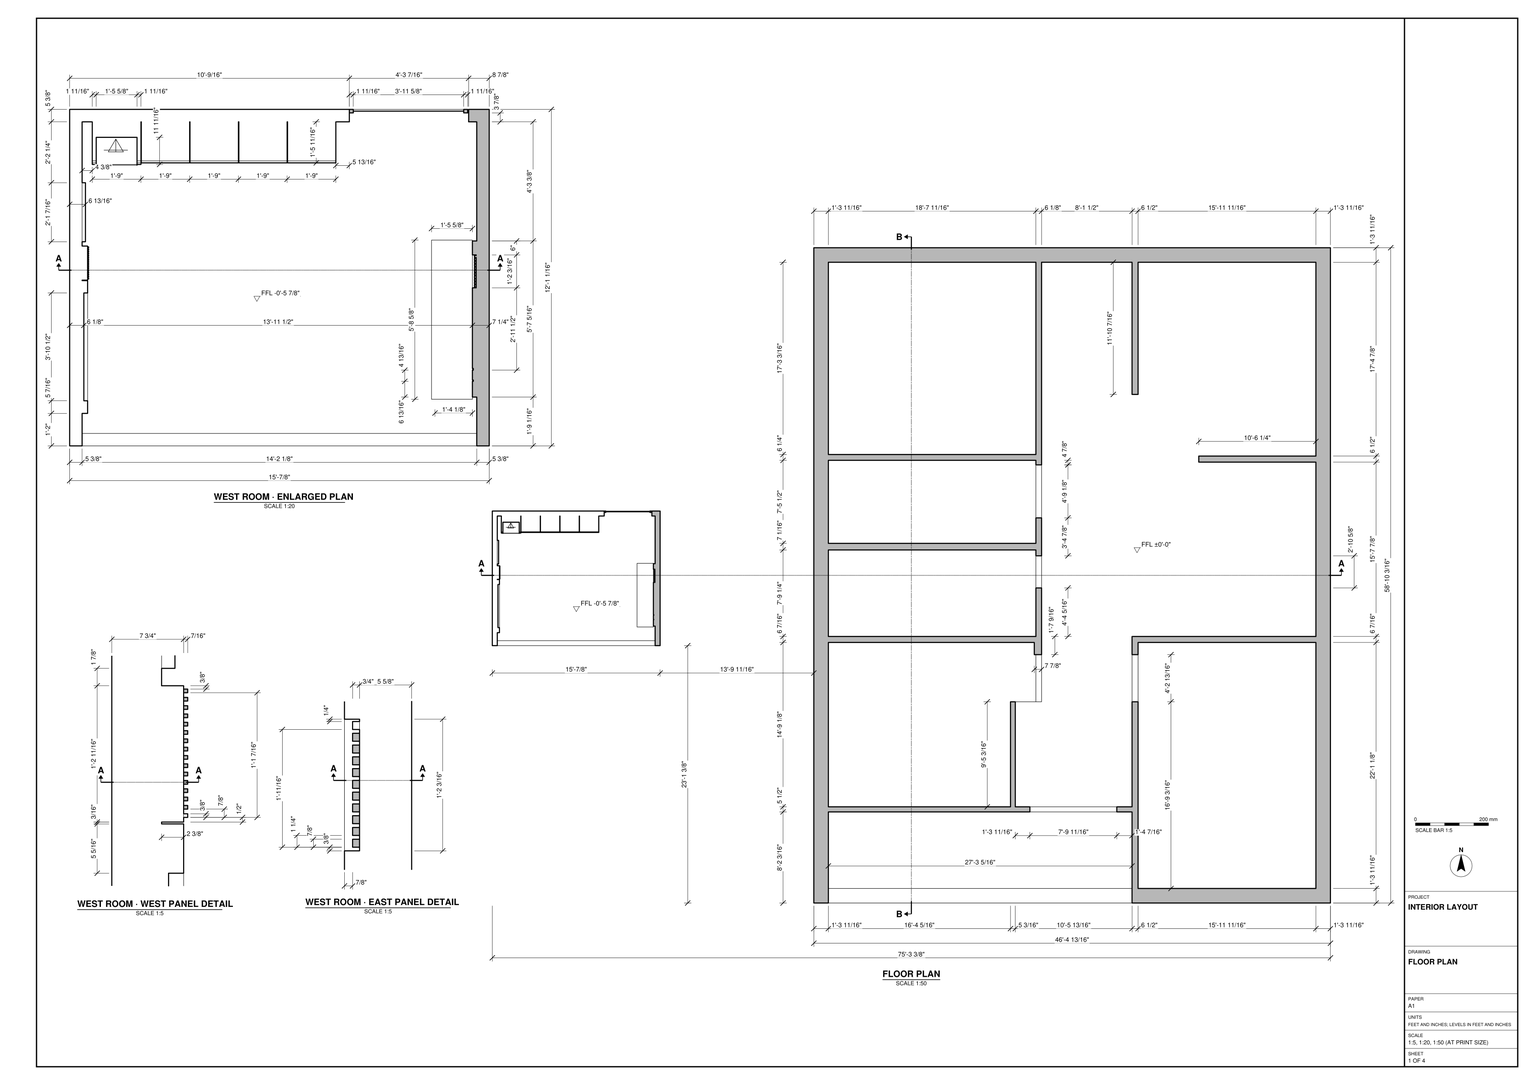
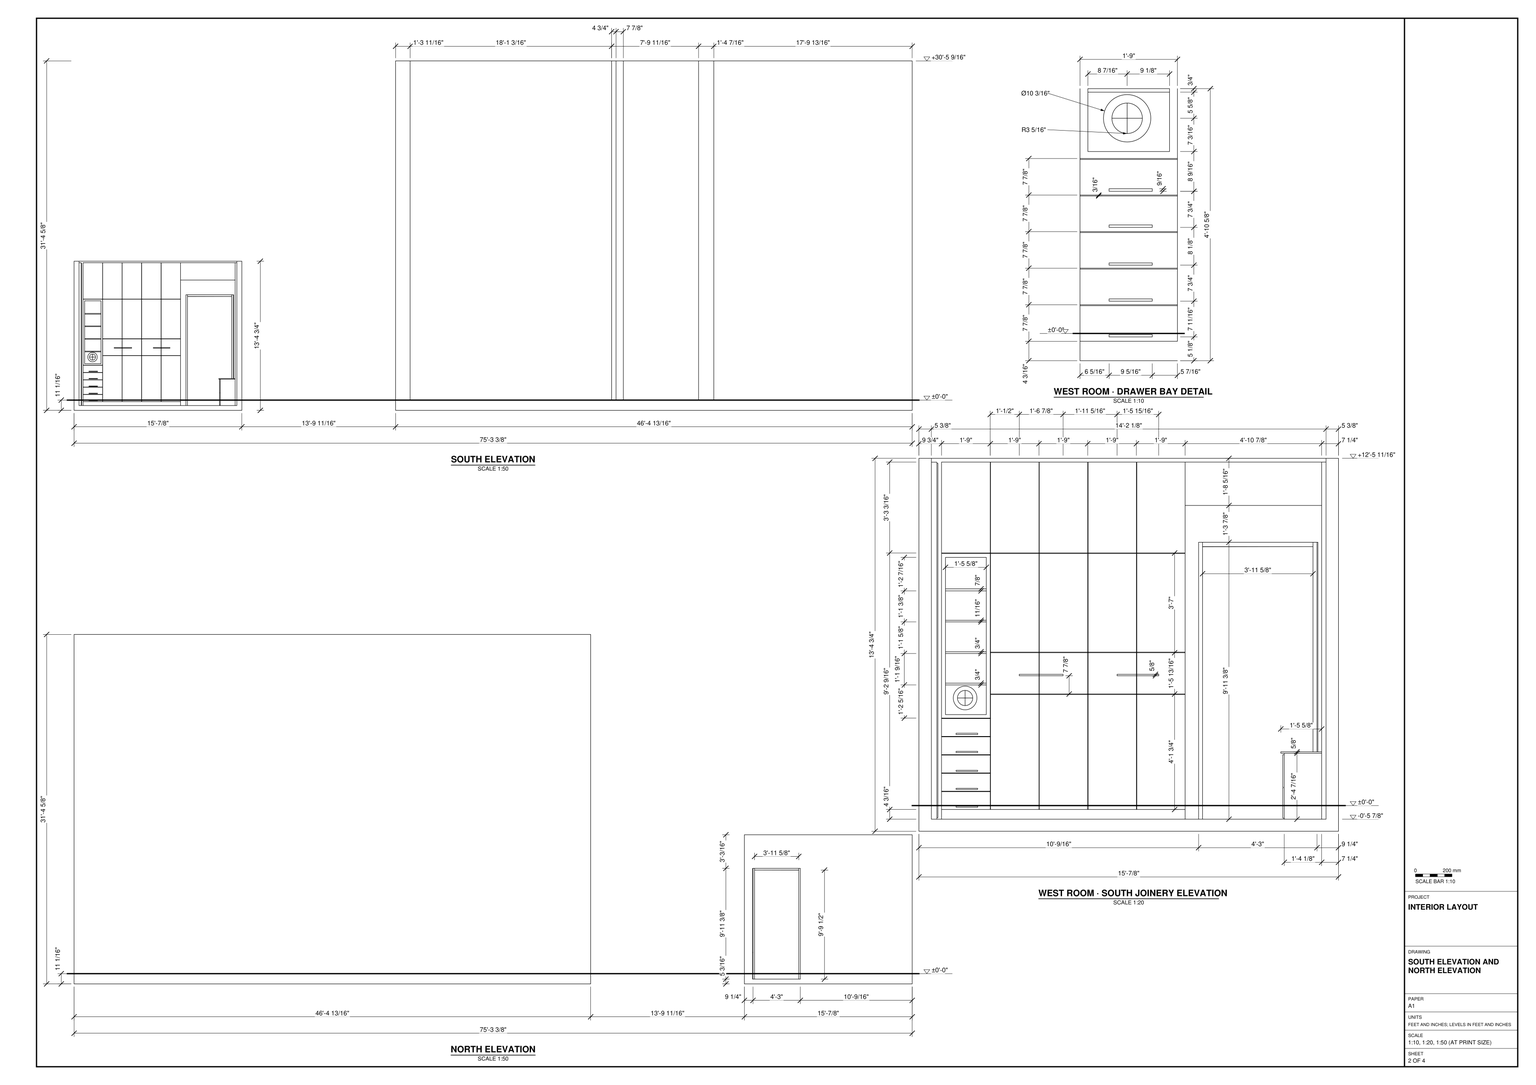
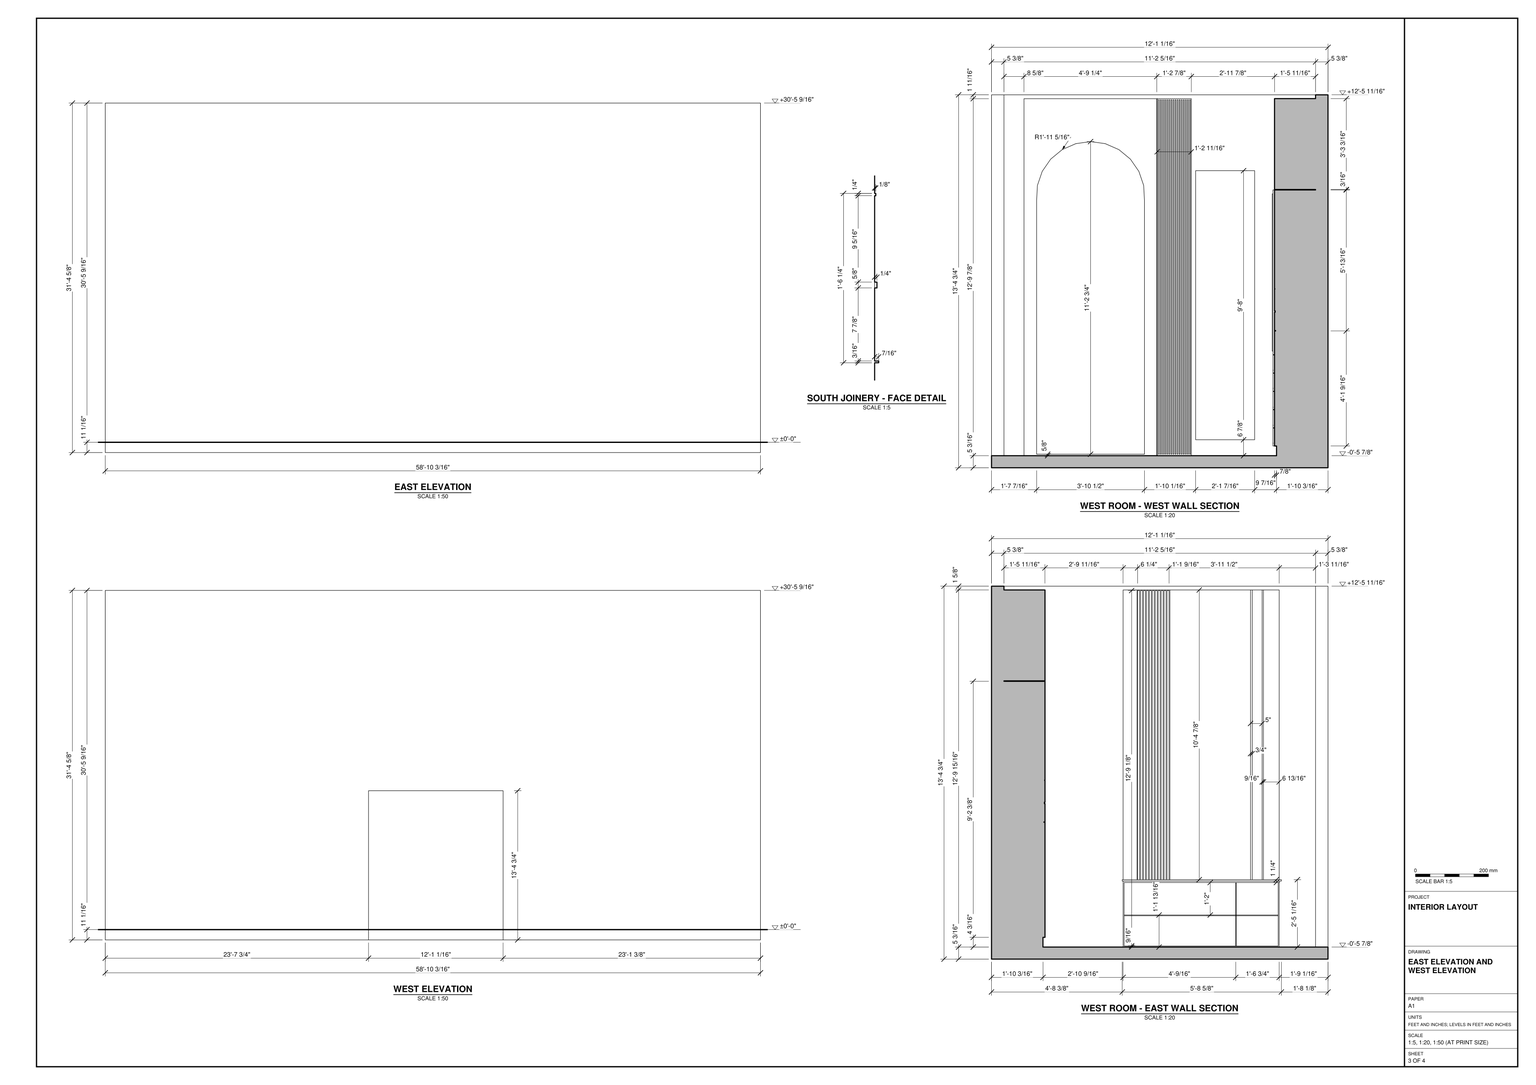
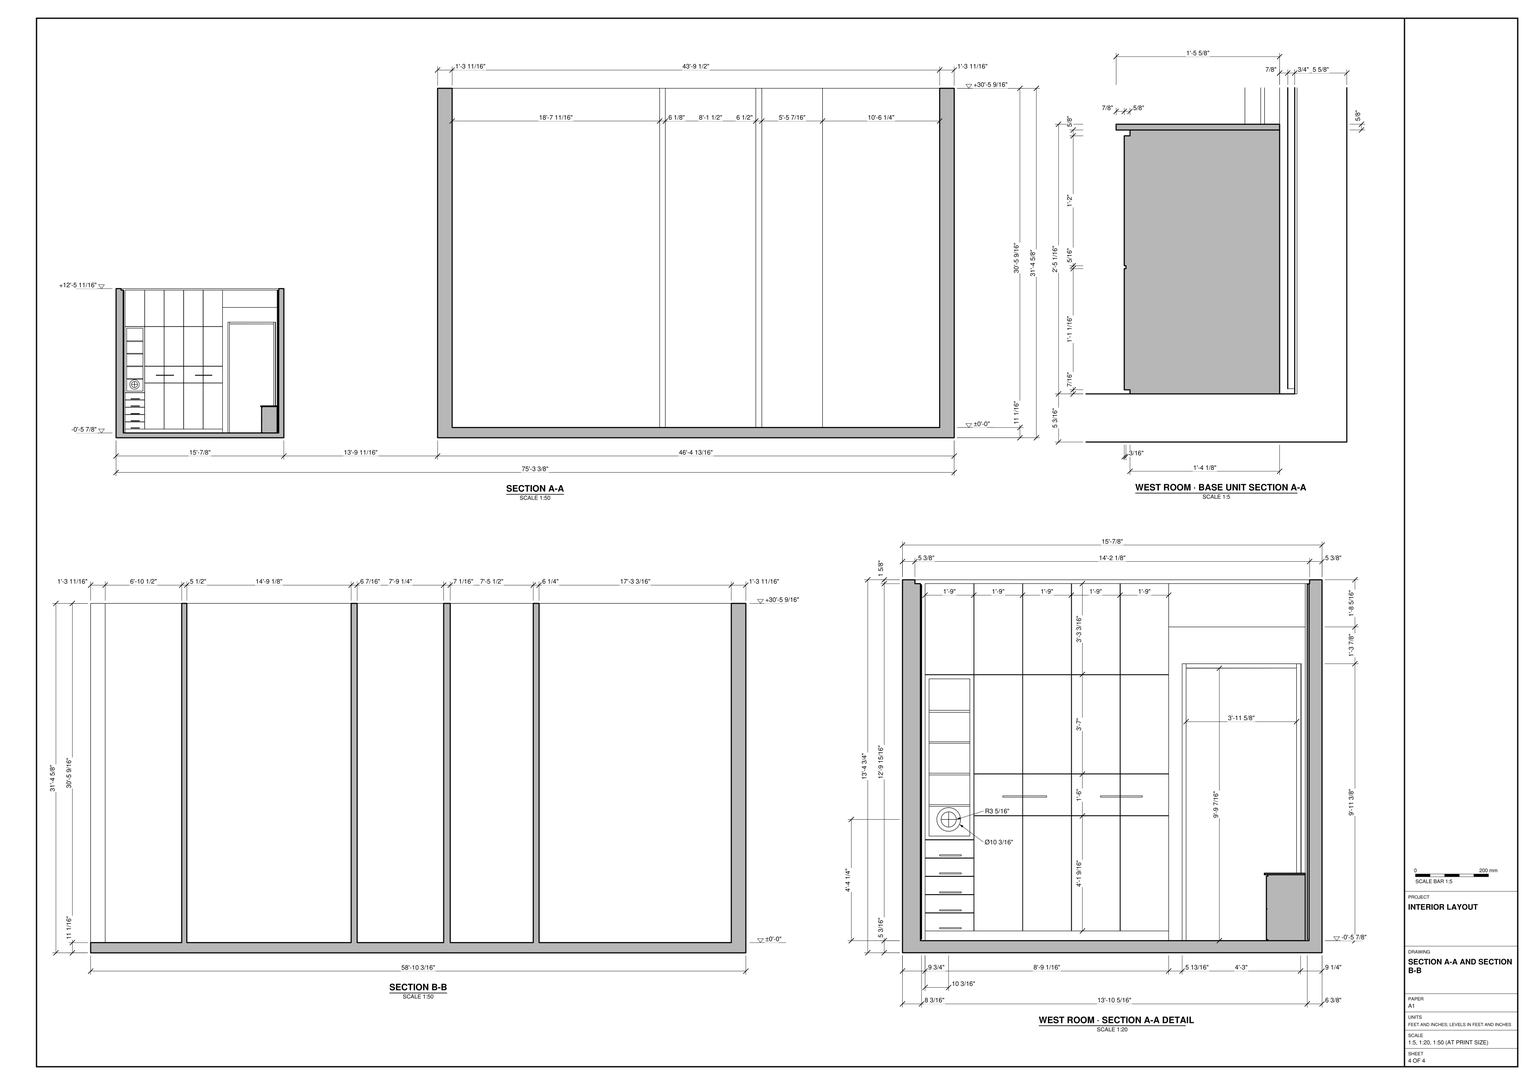
Work in feet and inches to model the layout in task_files/diagram_01.pdf. The overall model measures 75'-3 3/8" along X, 58'-10 3/16" along Y and 31'-4 5/8" along Z. Use ±0'-0" as the main ground-floor level. Set the detached west room at its lower finished floor level of -0'-5 7/8" and align it with the section line through the main block.

Model the floor slabs, perimeter walls and internal partitions at the thicknesses shown. In the main block, lay out the row of rooms along the west side and the larger spaces to the east. Preserve the passage openings, the short partition returns and the open stretch along the south edge. Use the elevations to establish the height difference between the main block and the west room.

Use the enlarged plan, joinery elevation and wall sections to fit out the west room. Model the full-height cabinet fronts, the narrow shelf and drawer bay with its circular inset, and the framed opening beside the cabinets. Distinguish the arched feature and ribbed panel on the west wall from the low cabinet and tall panels on the east wall. Decor and loose items may be any suitable library components. Keep shell elements and individual furniture or joinery pieces in separate groups or components, and use components for repeated parts. Save one SketchUp model as output_files/partitioned_interior_and_detached_west_room.skp.

# SketchUp Ruby script. Lengths in inches.
U = 1.inch
M = Sketchup.active_model
def pt(a) = Geom::Point3d.new(a.map { |v| v * U })
def face(e, loops, mat)
  f = e.add_face(loops[0].map { |a| pt(a) })
  loops[1..].each { |l| e.add_face(l.map { |a| pt(a) }).erase! }
  f.material = f.back_material = mat if mat
  f
end
# faces: each face lists its corners as indices into pts; further lists are holes
def faces(e, pts, list, mat = nil) = list.each { |f| face(e, (f[0].is_a?(Array) ? f : [f]).map { |l| l.map { |i| pts[i] } }, mat) }
# xy, xz, yz: faces in a plane at the given z, y or x. An outline is a flat list of corners, or four numbers for a rectangle; further outlines are holes
def ring(l) = l.size == 4 ? [[l[0], l[1]], [l[2], l[1]], [l[2], l[3]], [l[0], l[3]]] : l.each_slice(2).to_a
def flat(e, list, mat, &to3) = list.each { |f| face(e, (f[0].is_a?(Array) ? f : [f]).map { |l| ring(l).map { |u, v| to3.(u, v) } }, mat) }
def xy(e, z, list, mat = nil) = flat(e, list, mat) { |x, y| [x, y, z] }
def xz(e, y, list, mat = nil) = flat(e, list, mat) { |x, z| [x, y, z] }
def yz(e, x, list, mat = nil) = flat(e, list, mat) { |y, z| [x, y, z] }
def lines(e, pts, list) = list.each { |a, b| e.add_line(pt(pts[a]), pt(pts[b])) }
# prism: a flat outline (further loops are holes) pulled along v
def prism(e, loops, v, mat = nil)
  f = face(e, loops, mat); d = Geom::Vector3d.new(v.map { |x| x * U })
  f.pushpull(f.normal.samedirection?(d) ? d.length : -d.length)
end
def box(e, o, s, mat = nil) = prism(e, [[o, [o[0] + s[0], o[1], o[2]], [o[0] + s[0], o[1] + s[1], o[2]], [o[0], o[1] + s[1], o[2]]]], [0, 0, s[2]], mat)
def at(x, y, z, deg = 0) = Geom::Transformation.translation(pt([x, y, z])) * Geom::Transformation.rotation(ORIGIN, Z_AXIS, deg.degrees)
def axes(o, x, y, z) = Geom::Transformation.new([*x, 0, *y, 0, *z, 0, *pt(o).to_a, 1])
def part(name) = M.definitions.add(name)
# library, detail: a bought-in or finely detailed component or shape, given as its bounding box
def library(name, o, s) = part(name).tap { |d| box(d.entities, o, s) }
def detail(e, o, s) = box(e.add_group.entities, o, s)
def put(e, d, t, mat = nil) = e.add_instance(d, t).tap { |i| i.material = mat if mat }
def group(e, t, mat = nil) = e.add_group.tap { |g| g.transformation = t; g.material = mat if mat }.entities
root = M.entities
M.materials.add("Polis06_194").color = [79, 50, 36]
M.materials.add("[0009_Linen]").color = [250, 240, 230]
M.materials.add("[0029_BlanchedAlmond]").color = [255, 235, 205]
M.materials.add("[0035_Tan]").color = [210, 180, 140]
M.materials.add("[0133_Gray]").color = [190, 168, 135]
M.materials.add("[0136_Charcoal]").color = [35, 35, 35]
M.materials.add("[0137_Black]").color = [0, 0, 0]
M.materials.add("[Carrera Marble]").color = [207, 207, 207]
M.materials.add("[Mirror 02]").color = [229, 229, 229]
M.materials.add("[Translucent Glass Gray]").color = [128, 128, 128]
M.materials["[Translucent Glass Gray]"].alpha = 0.5
M.materials.add("[Wood Cherry Original]").color = [152, 86, 42]
c1 = part("Interior door")
xy(c1.entities,0,[[0,0,4.72,1.18],[0,34.25,4.72,35.43]],"Polis06_194")
xy(c1.entities,85.26,[[0,1.18,4.72,34.25]],"Polis06_194")
xy(c1.entities,86.61,[[0,0,4.72,35.43]],"Polis06_194")
xz(c1.entities,0,[[0,0,4.72,86.61]],"Polis06_194")
xz(c1.entities,1.18,[[0,0,2.36,85.26],[2.36,0,4.72,85.26]],"Polis06_194")
xz(c1.entities,34.25,[[0,0,4.72,85.26]],"Polis06_194")
xz(c1.entities,35.43,[[0,0,4.72,86.61]],"Polis06_194")
yz(c1.entities,0,[[0,0,1.18,86.61],[34.25,0,35.43,86.61],[1.18,85.26,34.25,86.61]],"Polis06_194")
yz(c1.entities,2.36,[[1.18,0,34.25,0,34.25,85.21,1.18,85.26]],"Polis06_194")
yz(c1.entities,4.72,[[0,0,1.18,86.61],[34.25,0,35.43,86.61],[1.18,85.26,34.25,86.61]],"Polis06_194")
c2 = library("Spot Light\#1",[-5.1,-5.1,-11.05],[10.2,10.2,11.05])
xy(root,0,[[346.55,0,903.36,706.1875]])
xy(root,5.1875,[[157.51,298.4,173.63,365.69]])
xy(root,5.625,[[156.88,317.13,157.51,365.26]])
xy(root,5.625,[[156.88,298.84,157.51,316.93]],"[0137_Black]")
xy(root,11.0625,[[362.21,0,689.53,15.66],[362.21,15.66,689.53,98.16],[696.03,15.66,887.7,280.79],[579.43,98.16,673.12,103.66],[362.21,103.66,558.53,103.66,558.53,216.85,585.9,216.85,585.9,267.66,584.15,267.66,584.15,280.79,362.21,280.79],
  [563.71,103.66,689.53,103.66,689.53,287.25,887.7,287.25,887.7,475.14,761.45,475.14,761.45,481.67,887.7,481.67,887.7,690.53,696.03,690.53,696.03,548.07,689.53,548.07,689.53,690.53,592.03,690.53,592.03,216.85,563.71,216.85],[585.9,216.85,592.03,267.66],[689.53,216.85,696.03,267.66],[362.21,287.25,585.9,380.49],[585.9,339.56,592.03,374.18],
  [362.21,387.58,585.9,477.08],[585.9,415.06,592.03,472.18],[362.21,483.35,585.9,690.53]])
xy(root,18.6875,[[156.88,298.84,157.07,316.93],[156.88,317.13,157.07,365.26]],"[0137_Black]")
xy(root,19,[[156.88,298.84,157.07,316.93],[156.88,317.13,157.07,365.26]],"[0137_Black]")
xy(root,33,[[156.88,298.84,157.51,316.93],[156.88,317.13,157.51,365.26]],"[0137_Black]")
xy(root,33.625,[[156.01,297.47,173.63,366.07]])
xy(root,34.25,[[156.01,297.47,173.63,366.07]],"[Wood Cherry Original]")
xy(root,50.27,[[11.44,398.37,29.04,398.68]],"[Translucent Glass Gray]")
xy(root,118.05,[[11.44,398.37,29.04,398.68]],"[Translucent Glass Gray]")
xy(root,376.625,[[346.55,0,362.21,0,362.21,98.16,579.43,98.16,579.43,103.66,563.71,103.66,563.71,216.85,558.53,216.85,558.53,103.66,362.21,103.66,362.21,280.79,584.15,280.79,584.15,267.66,592.03,267.66,592.03,339.56,585.9,339.56,585.9,287.25,362.21,287.25,362.21,690.53,887.7,690.53,887.7,481.67,761.45,481.67,761.45,475.14,887.7,475.14,887.7,15.66,696.03,15.66,696.03,216.85,689.53,216.85,689.53,103.66,673.12,103.66,673.12,98.16,689.53,98.16,689.53,0,903.36,0,903.36,706.1875,346.55,706.1875],[689.53,267.66,696.03,267.66,696.03,280.79,887.7,280.79,887.7,287.25,689.53,287.25],[585.9,374.18,592.03,374.18,592.03,415.06,585.9,415.06,585.9,387.58,362.21,387.58,362.21,380.49,585.9,380.49],[585.9,472.18,592.03,472.18,592.03,690.53,585.9,690.53,585.9,483.35,362.21,483.35,362.21,477.08,585.9,477.08],[689.53,548.07,696.03,690.53]])
xz(root,0,[[346.55,0,903.36,0,903.36,376.625,689.53,376.625,689.53,11.0625,362.21,11.0625,362.21,376.625,346.55,376.625]])
xz(root,15.66,[[696.03,11.0625,887.7,376.625]])
xz(root,98.16,[[362.21,11.0625,579.43,376.625],[673.12,11.0625,689.53,376.625]])
xz(root,103.66,[[362.21,11.0625,558.53,376.625],[563.71,11.0625,579.43,376.625],[673.12,11.0625,689.53,376.625]])
xz(root,216.85,[[558.53,11.0625,563.71,376.625],[689.53,11.0625,696.03,376.625]])
xz(root,267.66,[[584.15,11.0625,592.03,376.625],[689.53,11.0625,696.03,376.625]])
xz(root,280.79,[[362.21,11.0625,584.15,376.625],[696.03,11.0625,887.7,376.625]])
xz(root,287.25,[[362.21,11.0625,585.9,376.625],[689.53,11.0625,887.7,376.625]])
xz(root,297.47,[[156.01,33.625,173.63,34.25]],"[Wood Cherry Original]")
xz(root,298.84,[[156.88,5.625,157.51,5.625,157.51,33,156.88,33,156.88,19,157.07,19,157.07,18.6875,156.88,18.6875]],"[0137_Black]")
xz(root,316.93,[[156.88,5.625,156.88,18.6875,157.07,18.6875,157.07,19,156.88,19,156.88,33,157.51,33,157.51,5.625]],"[0137_Black]")
xz(root,317.13,[[156.88,5.625,157.51,5.625,157.51,33,156.88,33,156.88,19,157.07,19,157.07,18.6875,156.88,18.6875]],"[0137_Black]")
xz(root,339.56,[[585.9,11.0625,592.03,376.625]])
xz(root,365.26,[[156.88,5.625,157.51,18.6875],[157.07,18.6875,157.51,19.1875],[156.88,19,156.88,33,157.51,33,157.51,19.1875,157.07,19.1875,157.07,19]],"[0137_Black]")
xz(root,366.07,[[156.01,33.625,173.63,34.25]],"[Wood Cherry Original]")
xz(root,374.18,[[585.9,11.0625,592.03,376.625]])
xz(root,380.49,[[362.21,11.0625,585.9,376.625]])
xz(root,387.58,[[362.21,11.0625,585.9,376.625]])
xz(root,415.06,[[585.9,11.0625,592.03,376.625]])
xz(root,472.18,[[585.9,11.0625,592.03,376.625]])
xz(root,475.14,[[761.45,11.0625,887.7,376.625]])
xz(root,477.08,[[362.21,11.0625,585.9,376.625]])
xz(root,481.67,[[761.45,11.0625,887.7,376.625]])
xz(root,483.35,[[362.21,11.0625,585.9,376.625]])
xz(root,548.07,[[689.53,11.0625,696.03,376.625]])
xz(root,690.53,[[362.21,11.0625,585.9,376.625],[592.03,11.0625,689.53,376.625],[696.03,11.0625,887.7,376.625]])
xz(root,706.1875,[[346.55,0,903.36,376.625]])
yz(root,11.44,[[398.37,50.27,398.68,118.05]],"[Translucent Glass Gray]")
yz(root,29.04,[[398.37,50.27,398.68,118.05]],"[Translucent Glass Gray]")
yz(root,156.01,[[297.47,33.625,366.07,34.25]],"[Wood Cherry Original]")
yz(root,156.88,[[298.84,5.625,316.93,18.6875],[317.13,5.625,365.26,18.6875],[298.84,19,316.93,33],[317.13,19,365.26,33]],"[0029_BlanchedAlmond]")
yz(root,157.07,[[298.84,18.6875,316.93,19],[317.13,18.6875,365.26,19]],"[0137_Black]")
yz(root,173.63,[[298.4,5.1875,365.69,5.1875,365.69,33.625,366.07,33.625,366.07,34.25,297.47,34.25,297.47,33.625,298.4,33.625]])
yz(root,346.55,[[0,0,706.1875,376.625]])
yz(root,362.21,[[0,11.0625,15.66,376.625],[15.66,11.0625,98.16,376.625],[103.66,11.0625,280.79,376.625],[287.25,11.0625,380.49,376.625],[387.58,11.0625,477.08,376.625],
  [483.35,11.0625,690.53,376.625]])
yz(root,558.53,[[103.66,11.0625,216.85,376.625]])
yz(root,563.71,[[103.66,11.0625,216.85,376.625]])
yz(root,579.43,[[98.16,11.0625,103.66,376.625]])
yz(root,584.15,[[267.66,11.0625,280.79,376.625]])
yz(root,585.9,[[287.25,11.0625,339.56,376.625],[374.18,11.0625,380.49,376.625],[387.58,11.0625,415.06,376.625],[472.18,11.0625,477.08,376.625],[483.35,11.0625,690.53,376.625]])
yz(root,592.03,[[267.66,11.0625,339.56,376.625],[374.18,11.0625,415.06,376.625],[472.18,11.0625,690.53,376.625]])
yz(root,673.12,[[98.16,11.0625,103.66,376.625]])
yz(root,689.53,[[0,11.0625,15.66,376.625],[15.66,11.0625,98.16,376.625],[103.66,11.0625,216.85,376.625],[267.66,11.0625,287.25,376.625],[548.07,11.0625,690.53,376.625]])
yz(root,696.03,[[15.66,11.0625,216.85,376.625],[267.66,11.0625,280.79,376.625],[548.07,11.0625,690.53,376.625]])
yz(root,761.45,[[475.14,11.0625,481.67,376.625]])
yz(root,887.7,[[15.66,11.0625,280.79,376.625],[287.25,11.0625,475.14,376.625],[481.67,11.0625,690.53,376.625]])
yz(root,903.36,[[0,0,706.1875,376.625]])
put(root,c1,axes([171.59,420.91,5.1875],[0,0.32,0],[-1.44,0,0],[0,0,1.37824]))
g1 = group(root,at(0,277.36,0))
xy(g1,0,[[0,0,180.875,145.0625]])
xy(g1,5.1875,[[5.37,0,175.51,5.37],[5.37,5.37,175.51,5.37,175.51,21.04,173.63,21.04,173.63,27.83,174.01,27.83,174.01,28.4,173.63,28.4,173.63,32.65,174.01,32.65,174.01,33.4,173.63,33.4,173.63,68.15,175.26,68.15,175.26,82.33,173.63,82.33,173.63,88.33,175.51,88.33,175.51,139.7,172.01,139.7,172.01,145.0625,120.57,145.0625,120.57,139.7,114.76,139.7,114.76,122.88,9.74,122.88,9.74,139.7,5.37,139.7,5.37,86.13,7.74,86.13,7.74,71.45,5.37,71.45,5.37,71.25,7.74,71.25,7.74,14.01,5.37,14.01]])
xy(g1,5.75,[[174.51,81.23,175.26,82.08]])
xy(g1,5.84,[[7.74,71.95,8.18,72.34]])
xy(g1,9.375,[[30.87,122.01,51.75,122.88],[51.875,122.01,72.75,122.88],[72.9375,122.01,93.76,122.88],[93.94,122.01,114.76,122.88],[30.74,122.88,30.87,139.7],
  [51.75,122.88,51.875,139.7],[72.75,122.88,72.9375,139.7],[93.76,122.88,93.94,139.7]])
xy(g1,9.375,[[9.74,121.32,30.74,122.88]],"[0035_Tan]")
xy(g1,10.3125,[[16.01,121.32,25.32,121.38]])
xy(g1,10.8125,[[16.01,121.32,25.32,121.38]])
xy(g1,12.07,[[5.37,88.01,6.8,113.45]])
xy(g1,17.04,[[9.74,121.32,30.74,122.01]],"[0035_Tan]")
xy(g1,17.25,[[9.74,121.32,30.74,122.01]],"[0035_Tan]")
xy(g1,18.02,[[16.01,121.32,25.32,121.38]])
xy(g1,18.5,[[16.01,121.32,25.32,121.38]])
xy(g1,24.93,[[9.74,121.32,30.74,122.01]],"[0035_Tan]")
xy(g1,25.13,[[9.74,121.32,30.74,122.01]],"[0035_Tan]")
xy(g1,25.78,[[16.01,121.32,25.32,121.38]])
xy(g1,26.26,[[16.01,121.32,25.32,121.38]])
xy(g1,32.8125,[[9.74,121.32,30.74,122.01]],"[0035_Tan]")
xy(g1,33.01,[[9.74,121.32,30.74,122.01]],"[0035_Tan]")
xy(g1,33.92,[[16.01,121.32,25.32,121.38]])
xy(g1,34.45,[[16.01,121.32,25.32,121.38]])
xy(g1,40.69,[[9.74,121.32,30.74,122.01]],"[0035_Tan]")
xy(g1,40.89,[[9.74,121.32,30.74,122.01]],"[0035_Tan]")
xy(g1,41.7,[[16.01,121.32,25.32,121.38]])
xy(g1,42.26,[[16.01,121.32,25.32,121.38]])
xy(g1,48.57,[[9.74,121.32,30.74,122.01]],"[0035_Tan]")
xy(g1,48.77,[[9.74,121.32,30.74,122.01]])
xy(g1,50.27,[[11.44,121.32,29.04,133.01]])
xy(g1,58.96,[[30.87,122.01,51.75,122.45],[51.875,122.01,72.75,122.45],[72.9375,122.01,93.76,122.45],[93.94,122.01,114.76,122.45]],"[0029_BlanchedAlmond]")
xy(g1,59.15,[[30.87,122.01,51.75,122.45],[51.875,122.01,72.75,122.45],[72.9375,122.01,93.76,122.45],[93.94,122.01,114.76,122.45]],"[0029_BlanchedAlmond]")
xy(g1,63.07,[[11.44,121.32,29.04,133.01]],"[Carrera Marble]")
xy(g1,63.83,[[11.44,121.32,29.04,133.01]],"[Carrera Marble]")
xy(g1,67.02,[[43.25,122.01,51.75,122.2],[51.875,122.01,62.14,122.2],[85.42,122.01,93.76,122.26],[93.94,122.01,103.38,122.26]],"[0137_Black]")
xy(g1,67.65,[[43.25,122.01,51.75,122.2],[51.875,122.01,62.14,122.2],[85.42,122.01,93.76,122.26],[93.94,122.01,103.38,122.26]],"[0137_Black]")
xy(g1,76.62,[[11.44,121.32,29.04,133.01]],"[Carrera Marble]")
xy(g1,76.96,[[30.87,122.01,51.75,122.13],[51.875,122.01,72.75,122.13],[72.9375,122.01,93.76,122.13],[93.94,122.01,114.76,122.13]],"[0029_BlanchedAlmond]")
xy(g1,77.21,[[30.87,122.01,51.75,122.13],[51.875,122.01,72.75,122.13],[72.9375,122.01,93.76,122.13],[93.94,122.01,114.76,122.13]],"[0029_BlanchedAlmond]")
xy(g1,77.38,[[11.44,121.32,29.04,133.01]],"[Carrera Marble]")
xy(g1,90.24,[[11.44,121.32,29.04,133.01]],"[Carrera Marble]")
xy(g1,90.9375,[[11.44,121.32,29.04,133.01]])
xy(g1,103.61,[[11.44,121.32,29.04,133.01]],"[Carrera Marble]")
xy(g1,104.49,[[11.44,121.32,29.04,133.01]],"[Carrera Marble]")
xy(g1,118.05,[[11.44,121.32,29.04,133.01]],"[Carrera Marble]")
xy(g1,119.75,[[30.87,122.01,51.75,139.7],[51.875,122.01,72.75,139.7],[72.9375,122.01,93.76,139.7],[93.94,122.01,114.76,139.7]],"[0029_BlanchedAlmond]")
xy(g1,119.75,[[9.74,121.32,30.74,139.7]],"[0137_Black]")
xy(g1,119.9375,[[9.74,122.01,30.74,139.7],[30.87,122.01,51.75,139.7],[51.875,122.01,72.75,139.7],[72.9375,122.01,93.76,139.7],[93.94,122.01,114.76,139.7]],"[0035_Tan]")
xy(g1,124.5625,[[120.57,139.7,172.01,145.0625]])
xy(g1,128.0625,[[5.37,88.01,6.8,113.45]],"[Mirror 02]")
xy(g1,140.4375,[[114.76,136.63,175.51,139.7]])
xy(g1,158.59,[[7.74,71.95,8.18,72.34],[7.74,72.84,8.18,73.23],[7.74,73.74,8.18,74.13],[7.74,74.63,8.18,75.03],[7.74,75.53,8.18,75.92],
  [7.74,76.43,8.18,76.82],[7.74,77.32,8.18,77.71],[7.74,78.22,8.18,78.61],[7.74,79.11,8.18,79.51],[7.74,80.01,8.18,80.4],
  [7.74,80.9,8.18,81.3],[7.74,81.8,8.18,82.19],[7.74,82.7,8.18,83.09],[7.74,83.59,8.18,83.98],[7.74,84.49,8.18,84.88],
  [7.74,85.38,8.18,85.78]],"[Wood Cherry Original]")
xy(g1,159.09,[[5.37,71.45,7.74,86.13]],"[Carrera Marble]")
xy(g1,159.125,[[114.76,136.63,175.51,139.7]])
xy(g1,159.125,[[9.74,122.01,30.74,139.7],[30.87,122.01,51.75,139.7],[51.875,122.01,72.75,139.7],[72.9375,122.01,93.76,139.7],[93.94,122.01,114.76,139.7]],"[0035_Tan]")
xy(g1,160.75,[[0,0,5.37,0,5.37,139.7,175.51,139.7,175.51,0,180.875,0,180.875,145.0625,0,145.0625]])
xz(g1,0,[[0,0,180.875,0,180.875,160.75,175.51,160.75,175.51,5.1875,5.37,5.1875,5.37,160.75,0,160.75]])
xz(g1,71.45,[[5.37,5.1875,7.74,159.09]],"[Carrera Marble]")
xz(g1,71.95,[[7.74,5.84,8.18,158.59]],"[Wood Cherry Original]")
xz(g1,72.34,[[7.74,5.84,8.18,158.59]],"[Wood Cherry Original]")
xz(g1,72.84,[[7.74,5.84,8.18,158.59]],"[Wood Cherry Original]")
xz(g1,73.23,[[7.74,5.84,8.18,158.59]],"[Wood Cherry Original]")
xz(g1,73.74,[[7.74,5.84,8.18,158.59]],"[Wood Cherry Original]")
xz(g1,74.13,[[7.74,5.84,8.18,158.59]],"[Wood Cherry Original]")
xz(g1,74.63,[[7.74,5.84,8.18,158.59]],"[Wood Cherry Original]")
xz(g1,74.88,[[174.51,5.75,175.26,158.875]],"[Wood Cherry Original]")
xz(g1,75.03,[[7.74,5.84,8.18,158.59]],"[Wood Cherry Original]")
xz(g1,75.53,[[7.74,5.84,8.18,158.59]],"[Wood Cherry Original]")
xz(g1,75.92,[[7.74,5.84,8.18,158.59]],"[Wood Cherry Original]")
xz(g1,76.43,[[7.74,5.84,8.18,158.59]],"[Wood Cherry Original]")
xz(g1,76.82,[[7.74,5.84,8.18,158.59]],"[Wood Cherry Original]")
xz(g1,77.32,[[7.74,5.84,8.18,158.59]],"[Wood Cherry Original]")
xz(g1,77.71,[[7.74,5.84,8.18,158.59]],"[Wood Cherry Original]")
xz(g1,78.22,[[7.74,5.84,8.18,158.59]],"[Wood Cherry Original]")
xz(g1,78.61,[[7.74,5.84,8.18,158.59]],"[Wood Cherry Original]")
xz(g1,79.11,[[7.74,5.84,8.18,158.59]],"[Wood Cherry Original]")
xz(g1,79.51,[[7.74,5.84,8.18,158.59]],"[Wood Cherry Original]")
xz(g1,80.01,[[7.74,5.84,8.18,158.59]],"[Wood Cherry Original]")
xz(g1,80.4,[[7.74,5.84,8.18,158.59]],"[Wood Cherry Original]")
xz(g1,80.9,[[7.74,5.84,8.18,158.59]],"[Wood Cherry Original]")
xz(g1,81.3,[[7.74,5.84,8.18,158.59]],"[Wood Cherry Original]")
xz(g1,81.8,[[7.74,5.84,8.18,158.59]],"[Wood Cherry Original]")
xz(g1,82.19,[[7.74,5.84,8.18,158.59]],"[Wood Cherry Original]")
xz(g1,82.7,[[7.74,5.84,8.18,158.59]],"[Wood Cherry Original]")
xz(g1,83.09,[[7.74,5.84,8.18,158.59]],"[Wood Cherry Original]")
xz(g1,83.59,[[7.74,5.84,8.18,158.59]],"[Wood Cherry Original]")
xz(g1,83.98,[[7.74,5.84,8.18,158.59]],"[Wood Cherry Original]")
xz(g1,84.49,[[7.74,5.84,8.18,158.59]],"[Wood Cherry Original]")
xz(g1,84.88,[[7.74,5.84,8.18,158.59]],"[Wood Cherry Original]")
xz(g1,85.38,[[7.74,5.84,8.18,158.59]],"[Wood Cherry Original]")
xz(g1,85.78,[[7.74,5.84,8.18,158.59]],"[Wood Cherry Original]")
xz(g1,86.13,[[5.37,5.1875,7.74,159.09]],"[Carrera Marble]")
xz(g1,88.01,[[5.37,12.07,6.8,128.0625]],"[Mirror 02]")
xz(g1,113.45,[[5.37,12.07,6.8,128.0625]],"[Mirror 02]")
xz(g1,121.32,[[[9.74,9.375,30.74,17.04],[16.01,10.3125,25.32,10.8125]],[[9.74,17.25,30.74,24.93],[16.01,18.02,25.32,18.5]],[[9.74,25.13,30.74,32.8125],[16.01,25.78,25.32,26.26]],[[9.74,33.01,30.74,40.69],[16.01,33.92,25.32,34.45]],[[9.74,40.89,30.74,48.57],[16.01,41.7,25.32,42.26]]],"[0035_Tan]")
xz(g1,121.32,[[[9.74,48.77,30.74,119.75],[11.44,50.27,11.44,118.05,29.04,118.05,29.04,104.49,11.44,104.49,11.44,103.61,29.04,103.61,29.04,90.9375,11.44,90.9375,11.44,90.24,29.04,90.24,29.04,77.38,11.44,77.38,11.44,76.62,29.04,76.62,29.04,63.83,11.44,63.83,11.44,63.07,29.04,63.07,29.04,50.27]]],"[0136_Charcoal]")
xz(g1,121.38,[[16.01,10.3125,25.32,10.8125],[16.01,18.02,25.32,18.5],[16.01,25.78,25.32,26.26],[16.01,33.92,25.32,34.45],[16.01,41.7,25.32,42.26]])
xz(g1,122.01,[[9.74,48.57,30.74,48.77]])
xz(g1,122.01,[[30.87,9.375,51.75,58.96],[51.875,9.375,72.75,58.96],[72.9375,9.375,93.76,58.96],[93.94,9.375,114.76,58.96],[30.87,77.21,51.75,119.75],
  [51.875,77.21,72.75,119.75],[72.9375,77.21,93.76,119.75],[93.94,77.21,114.76,119.75]],"[0029_BlanchedAlmond]")
xz(g1,122.01,[[9.74,17.04,30.74,17.25],[9.74,24.93,30.74,25.13],[9.74,32.8125,30.74,33.01],[9.74,40.69,30.74,40.89],[9.74,119.9375,30.74,159.125],
  [30.87,119.9375,51.75,159.125],[51.875,119.9375,72.75,159.125],[72.9375,119.9375,93.76,159.125],[93.94,119.9375,114.76,159.125]],"[0035_Tan]")
xz(g1,122.01,[[30.87,59.15,51.75,59.15,51.75,67.02,43.25,67.02,43.25,67.65,51.75,67.65,51.75,76.96,30.87,76.96],[51.875,59.15,72.75,59.15,72.75,76.96,51.875,76.96,51.875,67.65,62.14,67.65,62.14,67.02,51.875,67.02],[72.9375,59.15,93.76,59.15,93.76,67.02,85.42,67.02,85.42,67.65,93.76,67.65,93.76,76.96,72.9375,76.96],[93.94,59.15,114.76,59.15,114.76,76.96,93.94,76.96,93.94,67.65,103.38,67.65,103.38,67.02,93.94,67.02]],"[Carrera Marble]")
xz(g1,122.13,[[30.87,76.96,51.75,77.21],[51.875,76.96,72.75,77.21],[72.9375,76.96,93.76,77.21],[93.94,76.96,114.76,77.21]],"[0029_BlanchedAlmond]")
xz(g1,122.2,[[43.25,67.02,51.75,67.65],[51.875,67.02,62.14,67.65]],"[0137_Black]")
xz(g1,122.26,[[85.42,67.02,93.76,67.65],[93.94,67.02,103.38,67.65]],"[0137_Black]")
xz(g1,122.45,[[30.87,58.96,51.75,59.15],[51.875,58.96,72.75,59.15],[72.9375,58.96,93.76,59.15],[93.94,58.96,114.76,59.15]],"[0029_BlanchedAlmond]")
xz(g1,122.88,[[9.74,5.1875,114.76,9.375]],"[0137_Black]")
xz(g1,133.01,[[11.44,50.27,29.04,63.07],[11.44,63.83,29.04,76.62],[11.44,77.38,29.04,90.24],[11.44,90.9375,29.04,103.61],[11.44,104.49,29.04,118.05]],"[Carrera Marble]")
xz(g1,136.63,[[114.76,140.4375,175.51,159.125]],"[0009_Linen]")
xz(g1,139.7,[[[5.37,5.1875,9.74,5.1875,9.74,119.75,30.74,119.75,30.74,9.375,30.87,9.375,30.87,119.75,51.75,119.75,51.75,9.375,51.875,9.375,51.875,119.75,72.75,119.75,72.75,9.375,72.9375,9.375,72.9375,119.75,93.76,119.75,93.76,9.375,93.94,9.375,93.94,119.75,114.76,119.75,114.76,5.1875,120.57,5.1875,120.57,124.5625,172.01,124.5625,172.01,5.1875,175.51,5.1875,175.51,140.4375,114.76,140.4375,114.76,119.9375,93.94,119.9375,93.94,159.125,175.51,159.125,175.51,160.75,5.37,160.75],[9.74,119.9375,30.74,159.125],[30.87,119.9375,51.75,159.125],[51.875,119.9375,72.75,159.125],[72.9375,119.9375,93.76,159.125]]],"[0009_Linen]")
xz(g1,145.0625,[[[0,0,180.875,160.75],[120.57,5.1875,172.01,124.5625]]],"[0029_BlanchedAlmond]")
yz(g1,0,[[0,0,145.0625,160.75]])
yz(g1,5.37,[[0,5.1875,5.37,160.75],[71.25,5.1875,71.45,159.09]])
yz(g1,5.37,[[[5.37,5.1875,14.01,5.1875,14.01,159.09,86.13,159.09,86.13,5.1875,139.7,5.1875,139.7,160.75,5.37,160.75],[88.01,12.07,113.45,128.0625]]],"[0009_Linen]")
yz(g1,6.8,[[88.01,12.07,113.45,128.0625]],"[Mirror 02]")
yz(g1,7.74,[[[71.45,5.1875,86.13,159.09],[71.95,5.84,72.34,158.59]]],"[Carrera Marble]")
yz(g1,8.18,[[71.95,5.84,72.34,158.59],[72.84,5.84,73.23,158.59],[73.74,5.84,74.13,158.59],[74.63,5.84,75.03,158.59],[75.53,5.84,75.92,158.59],
  [76.43,5.84,76.82,158.59],[77.32,5.84,77.71,158.59],[78.22,5.84,78.61,158.59],[79.11,5.84,79.51,158.59],[80.01,5.84,80.4,158.59],
  [80.9,5.84,81.3,158.59],[81.8,5.84,82.19,158.59],[82.7,5.84,83.09,158.59],[83.59,5.84,83.98,158.59],[84.49,5.84,84.88,158.59],
  [85.38,5.84,85.78,158.59]],"[Wood Cherry Original]")
yz(g1,9.74,[[122.88,5.1875,139.7,9.375],[139.7,47.71,122.01,48.57,122.01,48.77,139.7,48.13]])
yz(g1,9.74,[[121.32,9.375,121.32,17.04,122.01,17.04,122.01,17.25,121.32,17.25,121.32,24.93,122.01,24.93,122.01,25.13,121.32,25.13,121.32,32.8125,122.01,32.8125,122.01,33.01,121.32,33.01,121.32,40.69,122.01,40.69,122.01,40.89,121.32,40.89,121.32,48.57,122.01,48.57,139.7,47.71,139.7,9.375],[122.01,119.9375,139.7,159.125]],"[0035_Tan]")
yz(g1,9.74,[[139.7,48.13,122.01,48.77,121.32,48.77,121.32,119.75,139.7,119.75]],"[0136_Charcoal]")
yz(g1,11.44,[[121.32,50.27,133.01,63.07],[121.32,63.83,133.01,76.62],[121.32,77.38,133.01,90.24],[121.32,90.9375,133.01,103.61],[121.32,104.49,133.01,118.05]],"[Carrera Marble]")
yz(g1,16.01,[[121.32,10.3125,121.38,10.8125],[121.32,18.02,121.38,18.5],[121.32,25.78,121.38,26.26],[121.32,33.92,121.38,34.45],[121.32,41.7,121.38,42.26]])
yz(g1,25.32,[[121.32,10.3125,121.38,10.8125],[121.32,18.02,121.38,18.5],[121.32,25.78,121.38,26.26],[121.32,33.92,121.38,34.45],[121.32,41.7,121.38,42.26]])
yz(g1,29.04,[[121.32,63.07,133.01,63.83],[121.32,76.62,133.01,77.38],[121.32,90.24,133.01,90.9375],[121.32,103.61,133.01,104.49]])
yz(g1,29.04,[[121.32,50.27,133.01,63.07],[121.32,63.83,133.01,76.62],[121.32,77.38,133.01,90.24],[121.32,90.9375,133.01,103.61],[121.32,104.49,133.01,118.05]],"[Carrera Marble]")
yz(g1,30.74,[[122.01,48.57,139.7,48.77]])
yz(g1,30.74,[[121.32,9.375,139.7,9.375,139.7,48.57,121.32,48.57,121.32,40.89,122.01,40.89,122.01,40.69,121.32,40.69,121.32,33.01,122.01,33.01,122.01,32.8125,121.32,32.8125,121.32,25.13,122.01,25.13,122.01,24.93,121.32,24.93,121.32,17.25,122.01,17.25,122.01,17.04,121.32,17.04],[122.01,119.9375,139.7,159.125]],"[0035_Tan]")
yz(g1,30.74,[[121.32,48.77,139.7,119.75]],"[0136_Charcoal]")
yz(g1,30.87,[[122.01,9.375,122.01,58.96,122.45,58.96,122.45,59.15,122.01,59.15,122.01,76.96,122.13,76.96,122.13,77.21,122.01,77.21,122.01,119.75,139.7,119.75,139.7,9.375]],"[0029_BlanchedAlmond]")
yz(g1,30.87,[[122.01,119.9375,139.7,159.125]],"[0035_Tan]")
yz(g1,43.25,[[122.01,67.02,122.2,67.65]],"[0137_Black]")
yz(g1,51.75,[[122.01,9.375,139.7,9.375,139.7,119.75,122.01,119.75,122.01,77.21,122.13,77.21,122.13,76.96,122.01,76.96,122.01,67.65,122.2,67.65,122.2,67.02,122.01,67.02,122.01,59.15,122.45,59.15,122.45,58.96,122.01,58.96]],"[0029_BlanchedAlmond]")
yz(g1,51.75,[[122.01,119.9375,139.7,159.125]],"[0035_Tan]")
yz(g1,51.875,[[122.01,9.375,122.01,58.96,122.45,58.96,122.45,59.15,122.01,59.15,122.01,67.02,122.2,67.02,122.2,67.65,122.01,67.65,122.01,76.96,122.13,76.96,122.13,77.21,122.01,77.21,122.01,119.75,139.7,119.75,139.7,9.375]],"[0029_BlanchedAlmond]")
yz(g1,51.875,[[122.01,119.9375,139.7,159.125]],"[0035_Tan]")
yz(g1,62.14,[[122.01,67.02,122.2,67.65]],"[0137_Black]")
yz(g1,72.75,[[122.01,9.375,139.7,9.375,139.7,119.75,122.01,119.75,122.01,77.21,122.13,77.21,122.13,76.96,122.01,76.96,122.01,59.15,122.45,59.15,122.45,58.96,122.01,58.96]],"[0029_BlanchedAlmond]")
yz(g1,72.75,[[122.01,119.9375,139.7,159.125]],"[0035_Tan]")
yz(g1,72.9375,[[122.01,9.375,122.01,58.96,122.45,58.96,122.45,59.15,122.01,59.15,122.01,76.96,122.13,76.96,122.13,77.21,122.01,77.21,122.01,119.75,139.7,119.75,139.7,9.375]],"[0029_BlanchedAlmond]")
yz(g1,72.9375,[[122.01,119.9375,139.7,159.125]],"[0035_Tan]")
yz(g1,85.42,[[122.01,67.02,122.26,67.65]],"[0137_Black]")
yz(g1,93.76,[[122.01,9.375,139.7,9.375,139.7,119.75,122.01,119.75,122.01,77.21,122.13,77.21,122.13,76.96,122.01,76.96,122.01,67.65,122.26,67.65,122.26,67.02,122.01,67.02,122.01,59.15,122.45,59.15,122.45,58.96,122.01,58.96]],"[0029_BlanchedAlmond]")
yz(g1,93.76,[[122.01,119.9375,139.7,159.125]],"[0035_Tan]")
yz(g1,93.94,[[122.01,9.375,122.01,58.96,122.45,58.96,122.45,59.15,122.01,59.15,122.01,67.02,122.26,67.02,122.26,67.65,122.01,67.65,122.01,76.96,122.13,76.96,122.13,77.21,122.01,77.21,122.01,119.75,139.7,119.75,139.7,9.375]],"[0029_BlanchedAlmond]")
yz(g1,93.94,[[122.01,119.9375,139.7,159.125]],"[0035_Tan]")
yz(g1,103.38,[[122.01,67.02,122.26,67.65]],"[0137_Black]")
yz(g1,114.76,[[122.01,9.375,139.7,9.375,139.7,119.75,122.01,119.75,122.01,77.21,122.13,77.21,122.13,76.96,122.01,76.96,122.01,59.15,122.45,59.15,122.45,58.96,122.01,58.96]],"[0029_BlanchedAlmond]")
yz(g1,114.76,[[122.01,119.9375,139.7,119.9375,139.7,140.4375,136.63,140.4375,136.63,159.125,122.01,159.125]],"[0035_Tan]")
yz(g1,114.76,[[122.88,5.1875,139.7,9.375]],"[0137_Black]")
yz(g1,120.57,[[139.7,5.1875,145.0625,124.5625]])
yz(g1,172.01,[[139.7,5.1875,145.0625,124.5625]])
yz(g1,175.51,[[0,5.1875,5.37,160.75]])
yz(g1,175.51,[[5.37,5.1875,5.37,160.75,139.7,160.75,139.7,159.125,136.63,159.125,136.63,140.4375,139.7,140.4375,139.7,5.1875,88.33,5.1875,88.33,159.125,21.04,159.125,21.04,5.1875]],"[0009_Linen]")
yz(g1,180.875,[[0,0,145.0625,160.75]])
p = [[171.2,39.32,5.1875],[171.2,39.57,5.1875],[171.2,41.63,5.1875],[171.2,41.88,5.1875]]
lines(g1,p,[[0,1],[2,3]])
put(g1,c2,axes([19.9,132.26,57.44],[1,0,0],[0,0,-1],[0,0.5,0]))
g2 = group(g1,at(173.63,21.04,5.1875))
xy(g2,153.9375,[[0,0,1.875,0,1.875,47.1,0,47.1,0,12.35,0.375,12.35,0.375,11.6,0,11.6,0,7.35,0.375,7.35,0.375,6.79,0,6.79],[1.625,47.1,1.875,61.29],[0,61.29,1.875,67.29]],"[Carrera Marble]")
xz(g2,0,[[0,0,1.875,153.9375]],"[Carrera Marble]")
xz(g2,6.79,[[0,0,0.375,153.9375]],"[Wood Cherry Original]")
xz(g2,7.35,[[0,0,0.375,153.9375]],"[Wood Cherry Original]")
xz(g2,11.6,[[0,0,0.375,153.9375]],"[Wood Cherry Original]")
xz(g2,12.35,[[0,0,0.375,153.9375]],"[Wood Cherry Original]")
xz(g2,47.1,[[0,0,1.625,153.9375]])
xz(g2,61.29,[[0,0,1.625,153.9375]])
xz(g2,67.29,[[0,0,1.875,153.9375]],"[Carrera Marble]")
yz(g2,0,[[0,0,6.79,153.9375],[7.35,0,11.6,153.9375],[12.35,0,47.1,153.9375],[61.29,0,67.29,153.9375]],"[Carrera Marble]")
yz(g2,0.375,[[6.79,0,7.35,153.9375],[11.6,0,12.35,153.9375]],"[Wood Cherry Original]")
yz(g2,1.625,[[[47.1,0,61.29,153.9375],[60.18,0.5625,61.04,153.6875]]])
g3 = group(g1,at(174.51,68.54,5.75),"[Wood Cherry Original]")
xy(g3,153.125,[[0,0,0.75,0.86],[0,1.27,0.75,2.125],[0,2.54,0.75,3.4],[0,3.81,0.75,4.66],[0,5.08,0.75,5.93],
  [0,6.34,0.75,7.2],[0,7.61,0.75,8.47],[0,8.88,0.75,9.74],[0,10.15,0.75,11.01],[0,11.42,0.75,12.28],
  [0,12.6875,0.75,13.55]])
xz(g3,0,[[0,0,0.75,153.125]])
xz(g3,0.86,[[0,0,0.75,153.125]])
xz(g3,1.27,[[0,0,0.75,153.125]])
xz(g3,2.125,[[0,0,0.75,153.125]])
xz(g3,2.54,[[0,0,0.75,153.125]])
xz(g3,3.4,[[0,0,0.75,153.125]])
xz(g3,3.81,[[0,0,0.75,153.125]])
xz(g3,4.66,[[0,0,0.75,153.125]])
xz(g3,5.08,[[0,0,0.75,153.125]])
xz(g3,5.93,[[0,0,0.75,153.125]])
xz(g3,7.2,[[0,0,0.75,153.125]])
xz(g3,7.61,[[0,0,0.75,153.125]])
xz(g3,8.47,[[0,0,0.75,153.125]])
xz(g3,8.88,[[0,0,0.75,153.125]])
xz(g3,9.74,[[0,0,0.75,153.125]])
xz(g3,10.15,[[0,0,0.75,153.125]])
xz(g3,11.01,[[0,0,0.75,153.125]])
xz(g3,11.42,[[0,0,0.75,153.125]])
xz(g3,12.28,[[0,0,0.75,153.125]])
xz(g3,12.6875,[[0,0,0.75,153.125]])
xz(g3,13.55,[[0,0,0.75,153.125]])
yz(g3,0,[[0,0,0.86,153.125],[1.27,0,2.125,153.125],[2.54,0,3.4,153.125],[3.81,0,4.66,153.125],[5.08,0,5.93,153.125],
  [6.34,0,7.2,153.125],[7.61,0,8.47,153.125],[8.88,0,9.74,153.125],[10.15,0,11.01,153.125],[11.42,0,12.28,153.125],
  [12.6875,0,13.55,153.125]])
g4 = group(g1,at(5.37,14.01,5.1875))
xy(g4,0.65,[[0.75,5.4375,2.375,51.92]],"[Carrera Marble]")
xy(g4,153.9,[[0,0,2.375,57.24]],"[Carrera Marble]")
xz(g4,0,[[0,0,2.375,153.9]],"[Carrera Marble]")
xz(g4,5.4375,[[0.75,0.65,2.375,110.09]],"[Carrera Marble]")
xz(g4,51.92,[[0.75,0.65,2.375,110.09]],"[Carrera Marble]")
xz(g4,57.24,[[0,0,2.375,153.9]],"[Carrera Marble]")
yz(g4,2.375,[[[0,0,57.24,153.9],[5.4375,0.65,5.4375,110.09,5.78,116.5,7.85,122.57,11.5,127.85,16.45,131.9375,22.32,134.52,28.68,135.4,35.04,134.52,40.91,131.9375,45.86,127.85,49.51,122.57,51.59,116.5,51.92,110.09,51.92,0.65]]],"[Carrera Marble]")
p = [[2.375,5.78,116.5],[2.375,5.4375,110.09],[0.75,5.4375,110.09],[0.75,5.78,116.5],[2.375,51.92,110.09],[2.375,51.59,116.5],
  [0.75,51.59,116.5],[0.75,51.92,110.09],[2.375,7.85,122.57],[0.75,7.85,122.57],[2.375,49.51,122.57],[0.75,49.51,122.57],
  [2.375,11.5,127.85],[0.75,11.5,127.85],[2.375,45.86,127.85],[0.75,45.86,127.85],[2.375,16.45,131.9375],[0.75,16.45,131.9375],
  [2.375,40.91,131.9375],[0.75,40.91,131.9375],[2.375,22.32,134.52],[0.75,22.32,134.52],[2.375,35.04,134.52],[0.75,35.04,134.52],
  [2.375,28.68,135.4],[0.75,28.68,135.4]]
faces(g4,p,[[0,1,2,3],[4,5,6,7],[8,0,3,9],[5,10,11,6],[12,8,9,13],[10,14,15,11],[16,12,13,17],[14,18,19,15],
  [20,16,17,21],[18,22,23,19],[24,20,21,25],[22,24,25,23]],"[Carrera Marble]")
g5 = group(g1,at(6.12,19.45,5.84))
yz(g5,0,[[0,0,46.49,0,46.49,109.4375,46.15,115.85,44.08,121.92,40.43,127.2,35.48,131.29,29.6,133.87,23.24,134.75,16.89,133.87,11.01,131.29,6.0625,127.2,2.41,121.92,0.34,115.85,0,109.4375]],"[0133_Gray]")
g6 = group(root,at(157.51,298.4,5.1875))
xy(g6,28.4375,[[0,0,16.125,67.29]],"[0029_BlanchedAlmond]")
xz(g6,0,[[0,0,16.125,28.4375]],"[0029_BlanchedAlmond]")
xz(g6,67.29,[[0,0,16.125,28.4375]],"[0029_BlanchedAlmond]")
yz(g6,0,[[[0,0,67.29,28.4375],[18.73,0.4375,66.85,27.8125],[0.4375,0.4375,18.53,27.8125]]],"[0029_BlanchedAlmond]")
